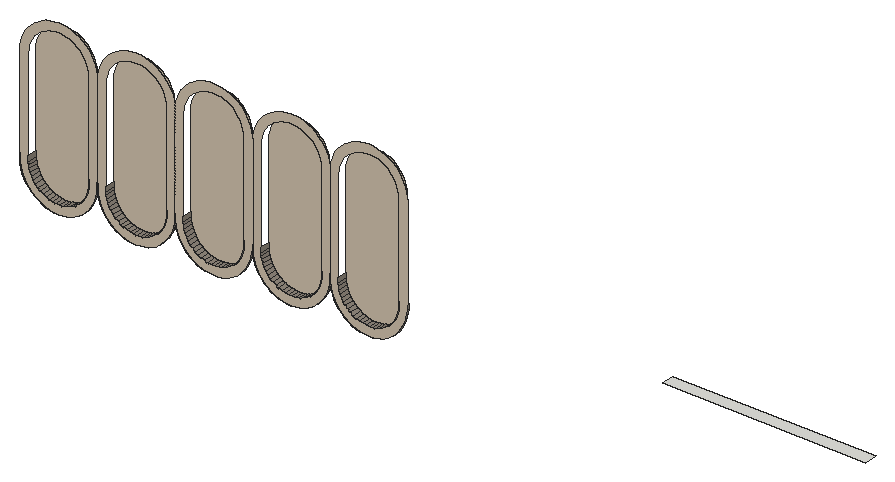
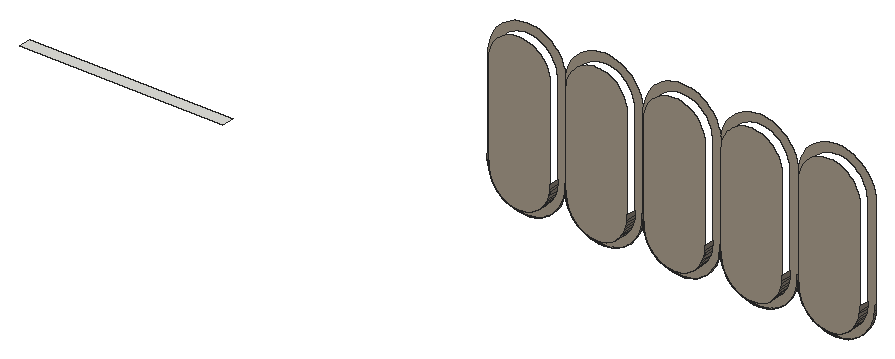
# SketchUp Ruby script. Lengths in inches.
U = 1.inch
M = Sketchup.active_model
def pt(a) = Geom::Point3d.new(a.map { |v| v * U })
def face(e, loops, mat)
  f = e.add_face(loops[0].map { |a| pt(a) })
  loops[1..].each { |l| e.add_face(l.map { |a| pt(a) }).erase! }
  f.material = f.back_material = mat if mat
  f
end
# faces: each face lists its corners as indices into pts; further lists are holes
def faces(e, pts, list, mat = nil) = list.each { |f| face(e, (f[0].is_a?(Array) ? f : [f]).map { |l| l.map { |i| pts[i] } }, mat) }
# xy, xz, yz: faces in a plane at the given z, y or x. An outline is a flat list of corners, or four numbers for a rectangle; further outlines are holes
def ring(l) = l.size == 4 ? [[l[0], l[1]], [l[2], l[1]], [l[2], l[3]], [l[0], l[3]]] : l.each_slice(2).to_a
def flat(e, list, mat, &to3) = list.each { |f| face(e, (f[0].is_a?(Array) ? f : [f]).map { |l| ring(l).map { |u, v| to3.(u, v) } }, mat) }
def xy(e, z, list, mat = nil) = flat(e, list, mat) { |x, y| [x, y, z] }
def xz(e, y, list, mat = nil) = flat(e, list, mat) { |x, z| [x, y, z] }
def yz(e, x, list, mat = nil) = flat(e, list, mat) { |y, z| [x, y, z] }
def lines(e, pts, list) = list.each { |a, b| e.add_line(pt(pts[a]), pt(pts[b])) }
# prism: a flat outline (further loops are holes) pulled along v
def prism(e, loops, v, mat = nil)
  f = face(e, loops, mat); d = Geom::Vector3d.new(v.map { |x| x * U })
  f.pushpull(f.normal.samedirection?(d) ? d.length : -d.length)
end
def box(e, o, s, mat = nil) = prism(e, [[o, [o[0] + s[0], o[1], o[2]], [o[0] + s[0], o[1] + s[1], o[2]], [o[0], o[1] + s[1], o[2]]]], [0, 0, s[2]], mat)
def at(x, y, z, deg = 0) = Geom::Transformation.translation(pt([x, y, z])) * Geom::Transformation.rotation(ORIGIN, Z_AXIS, deg.degrees)
def axes(o, x, y, z) = Geom::Transformation.new([*x, 0, *y, 0, *z, 0, *pt(o).to_a, 1])
def part(name) = M.definitions.add(name)
# library, detail: a bought-in or finely detailed component or shape, given as its bounding box
def library(name, o, s) = part(name).tap { |d| box(d.entities, o, s) }
def detail(e, o, s) = box(e.add_group.entities, o, s)
def put(e, d, t, mat = nil) = e.add_instance(d, t).tap { |i| i.material = mat if mat }
def group(e, t, mat = nil) = e.add_group.tap { |g| g.transformation = t; g.material = mat if mat }.entities
root = M.entities
M.materials.add("Heather_Band").color = [142, 133, 122]
M.materials.add("Lily_Blonde").color = [209, 194, 173]
xy(root,960.77,[[363.26,35.95,481.45,43.35]])
xz(root,3.89,[[[37.11,948.03,39.59,948.16,42.03,948.57,44.41,949.24,46.71,950.17,48.89,951.34,50.93,952.74,52.81,954.36,54.49,956.17,55.97,958.16,57.22,960.29,58.23,962.55,58.99,964.91,59.49,967.34,59.67,969.34,59.67,1026.72,59.5,1028.68,59,1031.11,58.24,1033.47,57.23,1035.73,55.98,1037.87,54.5,1039.86,52.82,1041.68,50.94,1043.3,48.9,1044.7,46.72,1045.875,44.42,1046.8,42.03,1047.47,39.59,1047.88,37.11,1048.02,34.64,1047.88,32.19,1047.47,29.81,1046.8,27.51,1045.875,25.33,1044.7,23.28,1043.3,21.41,1041.68,19.72,1039.86,18.24,1037.87,16.99,1035.73,15.98,1033.47,15.23,1031.11,14.73,1028.68,14.55,1026.72,14.55,969.34,14.74,967.34,15.23,964.91,15.99,962.55,17,960.29,18.26,958.16,19.73,956.17,21.42,954.36,23.3,952.74,25.34,951.34,27.52,950.17,29.8125,949.24,32.2,948.57,34.64,948.16],[37.11,952.88,35.17,952.99,33.25,953.3,31.38,953.83,29.58,954.56,27.86,955.48,26.26,956.58,24.79,957.85,23.46,959.28,22.3,960.84,21.32,962.51,20.52,964.29,19.93,966.14,19.54,968.05,19.4,969.5625,19.4,1026.5,19.53,1027.98,19.92,1029.88,20.51,1031.74,21.31,1033.52,22.29,1035.2,23.45,1036.76,24.78,1038.18,26.25,1039.46,27.85,1040.5625,29.57,1041.48,31.375,1042.21,33.25,1042.74,35.17,1043.06,37.11,1043.16,39.06,1043.06,40.98,1042.74,42.85,1042.21,44.66,1041.48,46.37,1040.5625,47.98,1039.46,49.45,1038.18,50.77,1036.76,51.9375,1035.2,52.92,1033.52,53.71,1031.74,54.31,1029.88,54.7,1027.98,54.83,1026.5,54.83,969.5625,54.69,968.05,54.3,966.14,53.71,964.29,52.91,962.51,51.93,960.84,50.77,959.28,49.44,957.85,47.97,956.58,46.36,955.48,44.65,954.56,42.85,953.83,40.97,953.3,39.06,952.99]]],"Lily_Blonde")
xz(root,4.02,[[[82.24,948.03,84.71,948.16,87.15,948.57,89.53,949.24,91.83,950.17,94.01,951.34,96.05,952.74,97.93,954.36,99.61,956.17,101.09,958.16,102.35,960.29,103.36,962.55,104.12,964.91,104.61,967.34,104.8,969.34,104.8,1026.72,104.62,1028.68,104.125,1031.11,103.37,1033.47,102.36,1035.73,101.1,1037.87,99.625,1039.86,97.9375,1041.68,96.0625,1043.3,94.02,1044.7,91.84,1045.875,89.54,1046.8,87.15,1047.47,84.71,1047.88,82.24,1048.02,79.76,1047.88,77.32,1047.47,74.93,1046.8,72.63,1045.875,70.45,1044.7,68.41,1043.3,66.53,1041.68,64.84,1039.86,63.37,1037.87,62.11,1035.73,61.1,1033.47,60.35,1031.11,59.85,1028.68,59.67,1026.72,59.72,1026.21,59.67,1023.73,59.67,972.28,59.72,969.8,59.67,969.34,59.86,967.34,60.36,964.91,61.11,962.55,62.125,960.29,63.38,958.16,64.86,956.17,66.54,954.36,68.42,952.74,70.46,951.34,72.64,950.17,74.9375,949.24,77.32,948.57,79.76,948.16],[82.24,952.88,80.29,952.99,78.375,953.3,76.5,953.83,74.7,954.56,72.98,955.48,71.38,956.58,69.91,957.85,68.58,959.28,67.42,960.84,66.4375,962.51,65.64,964.29,65.05,966.14,64.66,968.05,64.52,969.5625,64.52,1026.5,64.65,1027.98,65.04,1029.88,65.64,1031.74,66.43,1033.52,67.41,1035.2,68.57,1036.76,69.9,1038.18,71.37,1039.46,72.98,1040.5625,74.69,1041.48,76.5,1042.21,78.37,1042.74,80.29,1043.06,82.24,1043.16,84.18,1043.06,86.1,1042.74,87.97,1042.21,89.78,1041.48,91.49,1040.5625,93.1,1039.46,94.57,1038.18,95.9,1036.76,97.06,1035.2,98.04,1033.52,98.83,1031.74,99.43,1029.88,99.82,1027.98,99.95,1026.5,99.95,969.5625,99.8125,968.05,99.42,966.14,98.83,964.29,98.03,962.51,97.05,960.84,95.89,959.28,94.5625,957.85,93.09,956.58,91.49,955.48,89.77,954.56,87.97,953.83,86.1,953.3,84.18,952.99]],[[127.36,948.03,129.83,948.16,132.27,948.57,134.66,949.24,136.95,950.17,139.13,951.34,141.18,952.74,143.05,954.36,144.74,956.17,146.21,958.16,147.47,960.29,148.48,962.55,149.24,964.91,149.73,967.34,149.92,969.34,149.92,1026.72,149.74,1028.68,149.25,1031.11,148.49,1033.47,147.48,1035.73,146.23,1037.87,144.75,1039.86,143.0625,1041.68,141.1875,1043.3,139.14,1044.7,136.96,1045.875,134.66,1046.8,132.28,1047.47,129.83,1047.88,127.36,1048.02,124.88,1047.88,122.4375,1047.47,120.05,1046.8,117.75,1045.875,115.57,1044.7,113.53,1043.3,111.65,1041.68,109.97,1039.86,108.49,1037.87,107.24,1035.73,106.23,1033.47,105.47,1031.11,104.98,1028.68,104.8,1026.72,104.84,1026.21,104.8,1023.73,104.8,972.28,104.84,969.8,104.8,969.34,104.98,967.34,105.48,964.91,106.24,962.55,107.25,960.29,108.5,958.16,109.98,956.17,111.66,954.36,113.54,952.74,115.58,951.34,117.76,950.17,120.06,949.24,122.44,948.57,124.88,948.16],[127.36,952.88,125.41,952.99,123.5,953.3,121.625,953.83,119.82,954.56,118.11,955.48,116.5,956.58,115.03,957.85,113.7,959.28,112.54,960.84,111.56,962.51,110.77,964.29,110.17,966.14,109.78,968.05,109.64,969.5625,109.64,1026.5,109.77,1027.98,110.16,1029.88,110.76,1031.74,111.55,1033.52,112.53,1035.2,113.7,1036.76,115.02,1038.18,116.49,1039.46,118.1,1040.5625,119.8125,1041.48,121.62,1042.21,123.49,1042.74,125.41,1043.06,127.36,1043.16,129.3,1043.06,131.22,1042.74,133.1,1042.21,134.9,1041.48,136.62,1040.5625,138.22,1039.46,139.69,1038.18,141.02,1036.76,142.18,1035.2,143.16,1033.52,143.96,1031.74,144.55,1029.88,144.9375,1027.98,145.07,1026.5,145.07,969.5625,144.93,968.05,144.54,966.14,143.95,964.29,143.15,962.51,142.17,960.84,141.01,959.28,139.68,957.85,138.21,956.58,136.61,955.48,134.9,954.56,133.09,953.83,131.22,953.3,129.3,952.99]],[[172.48,948.03,174.95,948.16,177.39,948.57,179.78,949.24,182.08,950.17,184.26,951.34,186.3,952.74,188.17,954.36,189.86,956.17,191.34,958.16,192.59,960.29,193.6,962.55,194.36,964.91,194.86,967.34,195.04,969.34,195.04,1026.72,194.86,1028.68,194.37,1031.11,193.61,1033.47,192.6,1035.73,191.35,1037.87,189.87,1039.86,188.18,1041.68,186.31,1043.3,184.27,1044.7,182.08,1045.875,179.78,1046.8,177.4,1047.47,174.95,1047.88,172.48,1048.02,170,1047.88,167.56,1047.47,165.17,1046.8,162.875,1045.875,160.69,1044.7,158.65,1043.3,156.78,1041.68,155.09,1039.86,153.61,1037.87,152.36,1035.73,151.35,1033.47,150.59,1031.11,150.1,1028.68,149.92,1026.72,149.96,1026.21,149.92,1023.73,149.92,972.28,149.96,969.8,149.92,969.34,150.1,967.34,150.6,964.91,151.36,962.55,152.37,960.29,153.62,958.16,155.1,956.17,156.79,954.36,158.66,952.74,160.7,951.34,162.88,950.17,165.18,949.24,167.5625,948.57,170.01,948.16],[172.48,952.88,170.54,952.99,168.62,953.3,166.74,953.83,164.94,954.56,163.23,955.48,161.625,956.58,160.15,957.85,158.83,959.28,157.67,960.84,156.68,962.51,155.89,964.29,155.29,966.14,154.9,968.05,154.76,969.5625,154.76,1026.5,154.9,1027.98,155.28,1029.88,155.88,1031.74,156.67,1033.52,157.66,1035.2,158.82,1036.76,160.14,1038.18,161.62,1039.46,163.22,1040.5625,164.93,1041.48,166.74,1042.21,168.61,1042.74,170.53,1043.06,172.48,1043.16,174.42,1043.06,176.34,1042.74,178.22,1042.21,180.02,1041.48,181.74,1040.5625,183.34,1039.46,184.82,1038.18,186.14,1036.76,187.3,1035.2,188.29,1033.52,189.08,1031.74,189.67,1029.88,190.0625,1027.98,190.2,1026.5,190.2,969.5625,190.06,968.05,189.67,966.14,189.07,964.29,188.28,962.51,187.29,960.84,186.13,959.28,184.81,957.85,183.33,956.58,181.73,955.48,180.02,954.56,178.21,953.83,176.34,953.3,174.42,952.99]],[[217.6,948.03,220.07,948.16,222.52,948.57,224.9,949.24,227.2,950.17,229.38,951.34,231.42,952.74,233.29,954.36,234.98,956.17,236.46,958.16,237.71,960.29,238.72,962.55,239.48,964.91,239.98,967.34,240.16,969.34,240.16,1026.72,239.98,1028.68,239.49,1031.11,238.73,1033.47,237.72,1035.73,236.47,1037.87,234.99,1039.86,233.3,1041.68,231.43,1043.3,229.39,1044.7,227.2,1045.875,224.91,1046.8,222.52,1047.47,220.08,1047.88,217.6,1048.02,215.125,1047.88,212.68,1047.47,210.3,1046.8,208,1045.875,205.8125,1044.7,203.77,1043.3,201.9,1041.68,200.21,1039.86,198.73,1037.87,197.48,1035.73,196.47,1033.47,195.71,1031.11,195.22,1028.68,195.04,1026.72,195.09,1026.21,195.04,1023.73,195.04,972.28,195.08,969.8,195.04,969.34,195.22,967.34,195.72,964.91,196.48,962.55,197.49,960.29,198.74,958.16,200.22,956.17,201.91,954.36,203.78,952.74,205.82,951.34,208,950.17,210.3,949.24,212.69,948.57,215.13,948.16],[217.6,952.88,215.66,952.99,213.74,953.3,211.87,953.83,210.0625,954.56,208.35,955.48,206.75,956.58,205.27,957.85,203.95,959.28,202.79,960.84,201.8,962.51,201.01,964.29,200.41,966.14,200.02,968.05,199.88,969.5625,199.88,1026.5,200.02,1027.98,200.41,1029.88,201,1031.74,201.79,1033.52,202.78,1035.2,203.9375,1036.76,205.26,1038.18,206.74,1039.46,208.34,1040.5625,210.06,1041.48,211.86,1042.21,213.74,1042.74,215.66,1043.06,217.6,1043.16,219.54,1043.06,221.47,1042.74,223.34,1042.21,225.15,1041.48,226.86,1040.5625,228.46,1039.46,229.9375,1038.18,231.26,1036.76,232.42,1035.2,233.41,1033.52,234.2,1031.74,234.8,1029.88,235.18,1027.98,235.32,1026.5,235.32,969.5625,235.18,968.05,234.79,966.14,234.19,964.29,233.4,962.51,232.41,960.84,231.25,959.28,229.93,957.85,228.46,956.58,226.85,955.48,225.14,954.56,223.33,953.83,221.46,953.3,219.54,952.99]]],"Lily_Blonde")
xz(root,4.77,[[14.55,969.34,14.55,972.28,14.51,969.8],[59.67,969.34,59.72,969.8,59.67,972.28],[104.8,969.34,104.84,969.8,104.8,972.28],[149.92,969.34,149.96,969.8,149.92,972.28],[195.04,969.34,195.08,969.8,195.04,972.28]],"Heather_Band")
xz(root,9.67,[[37.11,952.88,39.06,952.99,40.97,953.3,42.85,953.83,44.65,954.56,46.36,955.48,47.97,956.58,49.44,957.85,50.77,959.28,51.93,960.84,52.91,962.51,53.71,964.29,54.3,966.14,54.69,968.05,54.83,969.5625,54.83,1026.5,54.7,1027.98,54.31,1029.88,53.71,1031.74,52.92,1033.52,51.9375,1035.2,50.77,1036.76,49.45,1038.18,47.98,1039.46,46.37,1040.5625,44.66,1041.48,42.85,1042.21,40.98,1042.74,39.06,1043.06,37.11,1043.16,35.17,1043.06,33.25,1042.74,31.375,1042.21,29.57,1041.48,27.85,1040.5625,26.25,1039.46,24.78,1038.18,23.45,1036.76,22.29,1035.2,21.31,1033.52,20.51,1031.74,19.92,1029.88,19.53,1027.98,19.4,1026.5,19.4,969.5625,19.54,968.05,19.93,966.14,20.52,964.29,21.32,962.51,22.3,960.84,23.46,959.28,24.79,957.85,26.26,956.58,27.86,955.48,29.58,954.56,31.38,953.83,33.25,953.3,35.17,952.99],[82.24,952.88,84.18,952.99,86.1,953.3,87.97,953.83,89.77,954.56,91.49,955.48,93.09,956.58,94.5625,957.85,95.89,959.28,97.05,960.84,98.03,962.51,98.83,964.29,99.42,966.14,99.8125,968.05,99.95,969.5625,99.95,1026.5,99.82,1027.98,99.43,1029.88,98.83,1031.74,98.04,1033.52,97.06,1035.2,95.9,1036.76,94.57,1038.18,93.1,1039.46,91.49,1040.5625,89.78,1041.48,87.97,1042.21,86.1,1042.74,84.18,1043.06,82.24,1043.16,80.29,1043.06,78.37,1042.74,76.5,1042.21,74.69,1041.48,72.98,1040.5625,71.37,1039.46,69.9,1038.18,68.57,1036.76,67.41,1035.2,66.43,1033.52,65.64,1031.74,65.04,1029.88,64.65,1027.98,64.52,1026.5,64.52,969.5625,64.66,968.05,65.05,966.14,65.64,964.29,66.4375,962.51,67.42,960.84,68.58,959.28,69.91,957.85,71.38,956.58,72.98,955.48,74.7,954.56,76.5,953.83,78.375,953.3,80.29,952.99],[127.36,952.88,129.3,952.99,131.22,953.3,133.09,953.83,134.9,954.56,136.61,955.48,138.21,956.58,139.68,957.85,141.01,959.28,142.17,960.84,143.15,962.51,143.95,964.29,144.54,966.14,144.93,968.05,145.07,969.5625,145.07,1026.5,144.9375,1027.98,144.55,1029.88,143.96,1031.74,143.16,1033.52,142.18,1035.2,141.02,1036.76,139.69,1038.18,138.22,1039.46,136.62,1040.5625,134.9,1041.48,133.1,1042.21,131.22,1042.74,129.3,1043.06,127.36,1043.16,125.41,1043.06,123.49,1042.74,121.62,1042.21,119.8125,1041.48,118.1,1040.5625,116.49,1039.46,115.02,1038.18,113.7,1036.76,112.53,1035.2,111.55,1033.52,110.76,1031.74,110.16,1029.88,109.77,1027.98,109.64,1026.5,109.64,969.5625,109.78,968.05,110.17,966.14,110.77,964.29,111.56,962.51,112.54,960.84,113.7,959.28,115.03,957.85,116.5,956.58,118.11,955.48,119.82,954.56,121.625,953.83,123.5,953.3,125.41,952.99],[172.48,952.88,174.42,952.99,176.34,953.3,178.21,953.83,180.02,954.56,181.73,955.48,183.33,956.58,184.81,957.85,186.13,959.28,187.29,960.84,188.28,962.51,189.07,964.29,189.67,966.14,190.06,968.05,190.2,969.5625,190.2,1026.5,190.0625,1027.98,189.67,1029.88,189.08,1031.74,188.29,1033.52,187.3,1035.2,186.14,1036.76,184.82,1038.18,183.34,1039.46,181.74,1040.5625,180.02,1041.48,178.22,1042.21,176.34,1042.74,174.42,1043.06,172.48,1043.16,170.53,1043.06,168.61,1042.74,166.74,1042.21,164.93,1041.48,163.22,1040.5625,161.62,1039.46,160.14,1038.18,158.82,1036.76,157.66,1035.2,156.67,1033.52,155.88,1031.74,155.28,1029.88,154.9,1027.98,154.76,1026.5,154.76,969.5625,154.9,968.05,155.29,966.14,155.89,964.29,156.68,962.51,157.67,960.84,158.83,959.28,160.15,957.85,161.625,956.58,163.23,955.48,164.94,954.56,166.74,953.83,168.62,953.3,170.54,952.99],[217.6,952.88,219.54,952.99,221.46,953.3,223.33,953.83,225.14,954.56,226.85,955.48,228.46,956.58,229.93,957.85,231.25,959.28,232.41,960.84,233.4,962.51,234.19,964.29,234.79,966.14,235.18,968.05,235.32,969.5625,235.32,1026.5,235.18,1027.98,234.8,1029.88,234.2,1031.74,233.41,1033.52,232.42,1035.2,231.26,1036.76,229.9375,1038.18,228.46,1039.46,226.86,1040.5625,225.15,1041.48,223.34,1042.21,221.47,1042.74,219.54,1043.06,217.6,1043.16,215.66,1043.06,213.74,1042.74,211.86,1042.21,210.06,1041.48,208.34,1040.5625,206.74,1039.46,205.26,1038.18,203.9375,1036.76,202.78,1035.2,201.79,1033.52,201,1031.74,200.41,1029.88,200.02,1027.98,199.88,1026.5,199.88,969.5625,200.02,968.05,200.41,966.14,201.01,964.29,201.8,962.51,202.79,960.84,203.95,959.28,205.27,957.85,206.75,956.58,208.35,955.48,210.0625,954.56,211.87,953.83,213.74,953.3,215.66,952.99]],"Lily_Blonde")
yz(root,14.55,[[3.89,969.34,4.77,972.28]],"Heather_Band")
yz(root,19.4,[[3.89,969.5625,9.67,972.28]],"Heather_Band")
yz(root,54.83,[[3.89,969.5625,9.67,972.28]],"Heather_Band")
yz(root,59.67,[[3.89,969.34,4.77,972.28]],"Heather_Band")
yz(root,64.52,[[4.02,969.5625,9.67,972.28]],"Heather_Band")
yz(root,99.95,[[4.02,969.5625,9.67,972.28]],"Heather_Band")
yz(root,104.8,[[4.02,969.34,4.77,972.28]],"Heather_Band")
yz(root,109.64,[[4.02,969.5625,9.67,972.28]],"Heather_Band")
yz(root,145.07,[[4.02,969.5625,9.67,972.28]],"Heather_Band")
yz(root,149.92,[[4.02,969.34,4.77,972.28]],"Heather_Band")
yz(root,154.76,[[4.02,969.5625,9.67,972.28]],"Heather_Band")
yz(root,190.2,[[4.02,969.5625,9.67,972.28]],"Heather_Band")
yz(root,195.04,[[4.02,969.34,4.77,972.28]],"Heather_Band")
yz(root,199.88,[[4.02,969.5625,9.67,972.28]],"Heather_Band")
yz(root,235.32,[[4.02,969.5625,9.67,972.28]],"Heather_Band")
yz(root,240.16,[[4.02,969.34,4.77,972.28]],"Heather_Band")
p = [[34.64,4.77,948.16],[37.11,4.77,948.03],[37.11,3.89,948.03],[34.64,3.89,948.16],[39.59,4.77,948.16],[39.59,3.89,948.16],
  [79.76,4.77,948.16],[82.24,4.77,948.03],[82.24,4.02,948.03],[79.76,4.02,948.16],[84.71,4.77,948.16],[84.71,4.02,948.16],
  [124.88,4.77,948.16],[127.36,4.77,948.03],[127.36,4.02,948.03],[124.88,4.02,948.16],[129.83,4.77,948.16],[129.83,4.02,948.16],
  [170.01,4.77,948.16],[172.48,4.77,948.03],[172.48,4.02,948.03],[170.01,4.02,948.16],[174.95,4.77,948.16],[174.95,4.02,948.16],
  [215.13,4.77,948.16],[217.6,4.77,948.03],[217.6,4.02,948.03],[215.13,4.02,948.16],[220.07,4.77,948.16],[220.07,4.02,948.16],
  [32.2,4.77,948.57],[32.2,3.89,948.57],[42.03,4.77,948.57],[42.03,3.89,948.57],[77.32,4.77,948.57],[77.32,4.02,948.57],
  [87.15,4.77,948.57],[87.15,4.02,948.57],[122.44,4.77,948.57],[122.44,4.02,948.57],[132.27,4.77,948.57],[132.27,4.02,948.57],
  [167.5625,4.77,948.57],[167.5625,4.02,948.57],[177.39,4.77,948.57],[177.39,4.02,948.57],[212.69,4.77,948.57],[212.69,4.02,948.57],
  [222.52,4.77,948.57],[222.52,4.02,948.57],[29.8125,4.77,949.24],[29.8125,3.89,949.24],[44.41,4.77,949.24],[44.41,3.89,949.24],
  [74.9375,4.77,949.24],[74.9375,4.02,949.24],[89.53,4.77,949.24],[89.53,4.02,949.24],[120.06,4.77,949.24],[120.06,4.02,949.24],
  [134.66,4.77,949.24],[134.66,4.02,949.24],[165.18,4.77,949.24],[165.18,4.02,949.24],[179.78,4.77,949.24],[179.78,4.02,949.24],
  [210.3,4.77,949.24],[210.3,4.02,949.24],[224.9,4.77,949.24],[224.9,4.02,949.24],[27.52,4.77,950.17],[27.52,3.89,950.17],
  [46.71,4.77,950.17],[46.71,3.89,950.17],[72.64,4.77,950.17],[72.64,4.02,950.17],[91.83,4.77,950.17],[91.83,4.02,950.17],
  [117.76,4.77,950.17],[117.76,4.02,950.17],[136.95,4.77,950.17],[136.95,4.02,950.17],[162.88,4.77,950.17],[162.88,4.02,950.17],
  [182.08,4.77,950.17],[182.08,4.02,950.17],[208,4.77,950.17],[208,4.02,950.17],[227.2,4.77,950.17],[227.2,4.02,950.17],
  [25.34,4.77,951.34],[25.34,3.89,951.34],[48.89,4.77,951.34],[48.89,3.89,951.34],[70.46,4.77,951.34],[70.46,4.02,951.34],
  [94.01,4.77,951.34],[94.01,4.02,951.34],[115.58,4.77,951.34],[115.58,4.02,951.34],[139.13,4.77,951.34],[139.13,4.02,951.34],
  [160.7,4.77,951.34],[160.7,4.02,951.34],[184.26,4.77,951.34],[184.26,4.02,951.34],[205.82,4.77,951.34],[205.82,4.02,951.34],
  [229.38,4.77,951.34],[229.38,4.02,951.34],[23.3,4.77,952.74],[23.3,3.89,952.74],[50.93,4.77,952.74],[50.93,3.89,952.74],
  [68.42,4.77,952.74],[68.42,4.02,952.74],[96.05,4.77,952.74],[96.05,4.02,952.74],[113.54,4.77,952.74],[113.54,4.02,952.74],
  [141.18,4.77,952.74],[141.18,4.02,952.74],[158.66,4.77,952.74],[158.66,4.02,952.74],[186.3,4.77,952.74],[186.3,4.02,952.74],
  [203.78,4.77,952.74],[203.78,4.02,952.74],[231.42,4.77,952.74],[231.42,4.02,952.74],[21.42,4.77,954.36],[21.42,3.89,954.36],
  [52.81,4.77,954.36],[52.81,3.89,954.36],[66.54,4.77,954.36],[66.54,4.02,954.36],[97.93,4.77,954.36],[97.93,4.02,954.36],
  [111.66,4.77,954.36],[111.66,4.02,954.36],[143.05,4.77,954.36],[143.05,4.02,954.36],[156.79,4.77,954.36],[156.79,4.02,954.36],
  [188.17,4.77,954.36],[188.17,4.02,954.36],[201.91,4.77,954.36],[201.91,4.02,954.36],[233.29,4.77,954.36],[233.29,4.02,954.36],
  [35.17,9.67,952.99],[35.17,3.89,952.99],[37.11,3.89,952.88],[37.11,9.67,952.88],[39.06,3.89,952.99],[39.06,9.67,952.99],
  [80.29,9.67,952.99],[80.29,4.02,952.99],[82.24,4.02,952.88],[82.24,9.67,952.88],[84.18,4.02,952.99],[84.18,9.67,952.99],
  [125.41,9.67,952.99],[125.41,4.02,952.99],[127.36,4.02,952.88],[127.36,9.67,952.88],[129.3,4.02,952.99],[129.3,9.67,952.99],
  [170.54,9.67,952.99],[170.54,4.02,952.99],[172.48,4.02,952.88],[172.48,9.67,952.88],[174.42,4.02,952.99],[174.42,9.67,952.99],
  [215.66,9.67,952.99],[215.66,4.02,952.99],[217.6,4.02,952.88],[217.6,9.67,952.88],[219.54,4.02,952.99],[219.54,9.67,952.99],
  [33.25,9.67,953.3],[33.25,3.89,953.3],[40.97,3.89,953.3],[40.97,9.67,953.3],[78.375,9.67,953.3],[78.375,4.02,953.3],
  [86.1,4.02,953.3],[86.1,9.67,953.3],[123.5,9.67,953.3],[123.5,4.02,953.3],[131.22,4.02,953.3],[131.22,9.67,953.3],
  [168.62,9.67,953.3],[168.62,4.02,953.3],[176.34,4.02,953.3],[176.34,9.67,953.3],[213.74,9.67,953.3],[213.74,4.02,953.3],
  [221.46,4.02,953.3],[221.46,9.67,953.3],[31.38,9.67,953.83],[31.38,3.89,953.83],[42.85,3.89,953.83],[42.85,9.67,953.83],
  [76.5,9.67,953.83],[76.5,4.02,953.83],[87.97,4.02,953.83],[87.97,9.67,953.83],[121.625,9.67,953.83],[121.625,4.02,953.83],
  [133.09,4.02,953.83],[133.09,9.67,953.83],[166.74,9.67,953.83],[166.74,4.02,953.83],[178.21,4.02,953.83],[178.21,9.67,953.83],
  [211.87,9.67,953.83],[211.87,4.02,953.83],[223.33,4.02,953.83],[223.33,9.67,953.83],[29.58,9.67,954.56],[29.58,3.89,954.56],
  [44.65,3.89,954.56],[44.65,9.67,954.56],[74.7,9.67,954.56],[74.7,4.02,954.56],[89.77,4.02,954.56],[89.77,9.67,954.56],
  [119.82,9.67,954.56],[119.82,4.02,954.56],[134.9,4.02,954.56],[134.9,9.67,954.56],[164.94,9.67,954.56],[164.94,4.02,954.56],
  [180.02,4.02,954.56],[180.02,9.67,954.56],[210.0625,9.67,954.56],[210.0625,4.02,954.56],[225.14,4.02,954.56],[225.14,9.67,954.56],
  [19.73,4.77,956.17],[19.73,3.89,956.17],[54.49,4.77,956.17],[54.49,3.89,956.17],[64.86,4.77,956.17],[64.86,4.02,956.17],
  [99.61,4.77,956.17],[99.61,4.02,956.17],[109.98,4.77,956.17],[109.98,4.02,956.17],[144.74,4.77,956.17],[144.74,4.02,956.17],
  [155.1,4.77,956.17],[155.1,4.02,956.17],[189.86,4.77,956.17],[189.86,4.02,956.17],[200.22,4.77,956.17],[200.22,4.02,956.17],
  [234.98,4.77,956.17],[234.98,4.02,956.17],[27.86,9.67,955.48],[27.86,3.89,955.48],[46.36,3.89,955.48],[46.36,9.67,955.48],
  [72.98,9.67,955.48],[72.98,4.02,955.48],[91.49,4.02,955.48],[91.49,9.67,955.48],[118.11,9.67,955.48],[118.11,4.02,955.48],
  [136.61,4.02,955.48],[136.61,9.67,955.48],[163.23,9.67,955.48],[163.23,4.02,955.48],[181.73,4.02,955.48],[181.73,9.67,955.48],
  [208.35,9.67,955.48],[208.35,4.02,955.48],[226.85,4.02,955.48],[226.85,9.67,955.48],[26.26,9.67,956.58],[26.26,3.89,956.58],
  [47.97,3.89,956.58],[47.97,9.67,956.58],[71.38,9.67,956.58],[71.38,4.02,956.58],[93.09,4.02,956.58],[93.09,9.67,956.58],
  [116.5,9.67,956.58],[116.5,4.02,956.58],[138.21,4.02,956.58],[138.21,9.67,956.58],[161.625,9.67,956.58],[161.625,4.02,956.58],
  [183.33,4.02,956.58],[183.33,9.67,956.58],[206.75,9.67,956.58],[206.75,4.02,956.58],[228.46,4.02,956.58],[228.46,9.67,956.58],
  [18.26,4.77,958.16],[18.26,3.89,958.16],[55.97,4.77,958.16],[55.97,3.89,958.16],[63.38,4.77,958.16],[63.38,4.02,958.16],
  [101.09,4.77,958.16],[101.09,4.02,958.16],[108.5,4.77,958.16],[108.5,4.02,958.16],[146.21,4.77,958.16],[146.21,4.02,958.16],
  [153.62,4.77,958.16],[153.62,4.02,958.16],[191.34,4.77,958.16],[191.34,4.02,958.16],[198.74,4.77,958.16],[198.74,4.02,958.16],
  [236.46,4.77,958.16],[236.46,4.02,958.16],[24.79,9.67,957.85],[24.79,3.89,957.85],[49.44,3.89,957.85],[49.44,9.67,957.85],
  [69.91,9.67,957.85],[69.91,4.02,957.85],[94.5625,4.02,957.85],[94.5625,9.67,957.85],[115.03,9.67,957.85],[115.03,4.02,957.85],
  [139.68,4.02,957.85],[139.68,9.67,957.85],[160.15,9.67,957.85],[160.15,4.02,957.85],[184.81,4.02,957.85],[184.81,9.67,957.85],
  [205.27,9.67,957.85],[205.27,4.02,957.85],[229.93,4.02,957.85],[229.93,9.67,957.85],[23.46,9.67,959.28],[23.46,3.89,959.28],
  [50.77,3.89,959.28],[50.77,9.67,959.28],[68.58,9.67,959.28],[68.58,4.02,959.28],[95.89,4.02,959.28],[95.89,9.67,959.28],
  [113.7,9.67,959.28],[113.7,4.02,959.28],[141.01,4.02,959.28],[141.01,9.67,959.28],[158.83,9.67,959.28],[158.83,4.02,959.28],
  [186.13,4.02,959.28],[186.13,9.67,959.28],[203.95,9.67,959.28],[203.95,4.02,959.28],[231.25,4.02,959.28],[231.25,9.67,959.28],
  [17,4.77,960.29],[17,3.89,960.29],[57.22,4.77,960.29],[57.22,3.89,960.29],[62.125,4.77,960.29],[62.125,4.02,960.29],
  [102.35,4.77,960.29],[102.35,4.02,960.29],[107.25,4.77,960.29],[107.25,4.02,960.29],[147.47,4.77,960.29],[147.47,4.02,960.29],
  [152.37,4.77,960.29],[152.37,4.02,960.29],[192.59,4.77,960.29],[192.59,4.02,960.29],[197.49,4.77,960.29],[197.49,4.02,960.29],
  [237.71,4.77,960.29],[237.71,4.02,960.29],[22.3,9.67,960.84],[22.3,3.89,960.84],[51.93,3.89,960.84],[51.93,9.67,960.84],
  [67.42,9.67,960.84],[67.42,4.02,960.84],[97.05,4.02,960.84],[97.05,9.67,960.84],[112.54,9.67,960.84],[112.54,4.02,960.84],
  [142.17,4.02,960.84],[142.17,9.67,960.84],[157.67,9.67,960.84],[157.67,4.02,960.84],[187.29,4.02,960.84],[187.29,9.67,960.84],
  [202.79,9.67,960.84],[202.79,4.02,960.84],[232.41,4.02,960.84],[232.41,9.67,960.84],[15.99,4.77,962.55],[15.99,3.89,962.55],
  [58.23,4.77,962.55],[58.23,3.89,962.55],[61.11,4.77,962.55],[61.11,4.02,962.55],[103.36,4.77,962.55],[103.36,4.02,962.55],
  [106.24,4.77,962.55],[106.24,4.02,962.55],[148.48,4.77,962.55],[148.48,4.02,962.55],[151.36,4.77,962.55],[151.36,4.02,962.55],
  [193.6,4.77,962.55],[193.6,4.02,962.55],[196.48,4.77,962.55],[196.48,4.02,962.55],[238.72,4.77,962.55],[238.72,4.02,962.55],
  [21.32,9.67,962.51],[21.32,3.89,962.51],[52.91,3.89,962.51],[52.91,9.67,962.51],[66.4375,9.67,962.51],[66.4375,4.02,962.51],
  [98.03,4.02,962.51],[98.03,9.67,962.51],[111.56,9.67,962.51],[111.56,4.02,962.51],[143.15,4.02,962.51],[143.15,9.67,962.51],
  [156.68,9.67,962.51],[156.68,4.02,962.51],[188.28,4.02,962.51],[188.28,9.67,962.51],[201.8,9.67,962.51],[201.8,4.02,962.51],
  [233.4,4.02,962.51],[233.4,9.67,962.51],[20.52,9.67,964.29],[20.52,3.89,964.29],[53.71,3.89,964.29],[53.71,9.67,964.29],
  [65.64,9.67,964.29],[65.64,4.02,964.29],[98.83,4.02,964.29],[98.83,9.67,964.29],[110.77,9.67,964.29],[110.77,4.02,964.29],
  [143.95,4.02,964.29],[143.95,9.67,964.29],[155.89,9.67,964.29],[155.89,4.02,964.29],[189.07,4.02,964.29],[189.07,9.67,964.29],
  [201.01,9.67,964.29],[201.01,4.02,964.29],[234.19,4.02,964.29],[234.19,9.67,964.29],[15.23,4.77,964.91],[15.23,3.89,964.91],
  [58.99,4.77,964.91],[58.99,3.89,964.91],[60.36,4.77,964.91],[60.36,4.02,964.91],[104.12,4.77,964.91],[104.12,4.02,964.91],
  [105.48,4.77,964.91],[105.48,4.02,964.91],[149.24,4.77,964.91],[149.24,4.02,964.91],[150.6,4.77,964.91],[150.6,4.02,964.91],
  [194.36,4.77,964.91],[194.36,4.02,964.91],[195.72,4.77,964.91],[195.72,4.02,964.91],[239.48,4.77,964.91],[239.48,4.02,964.91],
  [19.93,9.67,966.14],[19.93,3.89,966.14],[54.3,3.89,966.14],[54.3,9.67,966.14],[65.05,9.67,966.14],[65.05,4.02,966.14],
  [99.42,4.02,966.14],[99.42,9.67,966.14],[110.17,9.67,966.14],[110.17,4.02,966.14],[144.54,4.02,966.14],[144.54,9.67,966.14],
  [155.29,9.67,966.14],[155.29,4.02,966.14],[189.67,4.02,966.14],[189.67,9.67,966.14],[200.41,9.67,966.14],[200.41,4.02,966.14],
  [234.79,4.02,966.14],[234.79,9.67,966.14],[14.74,4.77,967.34],[14.74,3.89,967.34],[59.49,4.77,967.34],[59.49,3.89,967.34],
  [59.86,4.77,967.34],[59.86,4.02,967.34],[104.61,4.77,967.34],[104.61,4.02,967.34],[104.98,4.77,967.34],[104.98,4.02,967.34],
  [149.73,4.77,967.34],[149.73,4.02,967.34],[150.1,4.77,967.34],[150.1,4.02,967.34],[194.86,4.77,967.34],[194.86,4.02,967.34],
  [195.22,4.77,967.34],[195.22,4.02,967.34],[239.98,4.77,967.34],[239.98,4.02,967.34],[19.54,9.67,968.05],[19.54,3.89,968.05],
  [54.69,3.89,968.05],[54.69,9.67,968.05],[64.66,9.67,968.05],[64.66,4.02,968.05],[99.8125,4.02,968.05],[99.8125,9.67,968.05],
  [109.78,9.67,968.05],[109.78,4.02,968.05],[144.93,4.02,968.05],[144.93,9.67,968.05],[154.9,9.67,968.05],[154.9,4.02,968.05],
  [190.06,4.02,968.05],[190.06,9.67,968.05],[200.02,9.67,968.05],[200.02,4.02,968.05],[235.18,4.02,968.05],[235.18,9.67,968.05],
  [14.55,4.77,969.34],[14.55,3.89,969.34],[59.67,4.77,969.34],[59.67,4.02,969.34],[59.67,3.89,969.34],[104.8,4.77,969.34],
  [104.8,4.02,969.34],[149.92,4.77,969.34],[149.92,4.02,969.34],[195.04,4.77,969.34],[195.04,4.02,969.34],[240.16,4.77,969.34],
  [240.16,4.02,969.34],[19.4,9.67,969.5625],[19.4,3.89,969.5625],[54.83,3.89,969.5625],[54.83,9.67,969.5625],[64.52,9.67,969.5625],
  [64.52,4.02,969.5625],[99.95,4.02,969.5625],[99.95,9.67,969.5625],[109.64,9.67,969.5625],[109.64,4.02,969.5625],[145.07,4.02,969.5625],
  [145.07,9.67,969.5625],[154.76,9.67,969.5625],[154.76,4.02,969.5625],[190.2,4.02,969.5625],[190.2,9.67,969.5625],[199.88,9.67,969.5625],
  [199.88,4.02,969.5625],[235.32,4.02,969.5625],[235.32,9.67,969.5625],[59.72,4.77,969.8],[59.72,4.02,969.8],[104.84,4.77,969.8],
  [104.84,4.02,969.8],[149.96,4.77,969.8],[149.96,4.02,969.8],[195.08,4.77,969.8],[195.08,4.02,969.8],[59.67,4.77,972.28],
  [59.67,4.02,972.28],[104.8,4.77,972.28],[104.8,4.02,972.28],[149.92,4.77,972.28],[149.92,4.02,972.28],[195.04,4.77,972.28],
  [195.04,4.02,972.28]]
faces(root,p,[[0,1,2,3],[1,4,5,2],[6,7,8,9],[7,10,11,8],[12,13,14,15],[13,16,17,14],[18,19,20,21],[19,22,23,20],
  [24,25,26,27],[25,28,29,26],[30,0,3,31],[4,32,33,5],[34,6,9,35],[10,36,37,11],[38,12,15,39],[16,40,41,17],
  [42,18,21,43],[22,44,45,23],[46,24,27,47],[28,48,49,29],[50,30,31,51],[32,52,53,33],[54,34,35,55],[36,56,57,37],
  [58,38,39,59],[40,60,61,41],[62,42,43,63],[44,64,65,45],[66,46,47,67],[48,68,69,49],[70,50,51,71],[52,72,73,53],
  [74,54,55,75],[56,76,77,57],[78,58,59,79],[60,80,81,61],[82,62,63,83],[64,84,85,65],[86,66,67,87],[68,88,89,69],
  [90,70,71,91],[72,92,93,73],[94,74,75,95],[76,96,97,77],[98,78,79,99],[80,100,101,81],[102,82,83,103],[84,104,105,85],
  [106,86,87,107],[88,108,109,89],[110,90,91,111],[92,112,113,93],[114,94,95,115],[96,116,117,97],[118,98,99,119],[100,120,121,101],
  [122,102,103,123],[104,124,125,105],[126,106,107,127],[108,128,129,109],[130,110,111,131],[112,132,133,113],[134,114,115,135],[116,136,137,117],
  [138,118,119,139],[120,140,141,121],[142,122,123,143],[124,144,145,125],[146,126,127,147],[128,148,149,129],[150,151,152,153],[153,152,154,155],
  [156,157,158,159],[159,158,160,161],[162,163,164,165],[165,164,166,167],[168,169,170,171],[171,170,172,173],[174,175,176,177],[177,176,178,179],
  [180,181,151,150],[155,154,182,183],[184,185,157,156],[161,160,186,187],[188,189,163,162],[167,166,190,191],[192,193,169,168],[173,172,194,195],
  [196,197,175,174],[179,178,198,199],[200,201,181,180],[183,182,202,203],[204,205,185,184],[187,186,206,207],[208,209,189,188],[191,190,210,211],
  [212,213,193,192],[195,194,214,215],[216,217,197,196],[199,198,218,219],[220,221,201,200],[203,202,222,223],[224,225,205,204],[207,206,226,227],
  [228,229,209,208],[211,210,230,231],[232,233,213,212],[215,214,234,235],[236,237,217,216],[219,218,238,239],[240,130,131,241],[132,242,243,133],
  [244,134,135,245],[136,246,247,137],[248,138,139,249],[140,250,251,141],[252,142,143,253],[144,254,255,145],[256,146,147,257],[148,258,259,149],
  [260,261,221,220],[223,222,262,263],[264,265,225,224],[227,226,266,267],[268,269,229,228],[231,230,270,271],[272,273,233,232],[235,234,274,275],
  [276,277,237,236],[239,238,278,279],[280,281,261,260],[263,262,282,283],[284,285,265,264],[267,266,286,287],[288,289,269,268],[271,270,290,291],
  [292,293,273,272],[275,274,294,295],[296,297,277,276],[279,278,298,299],[300,240,241,301],[242,302,303,243],[304,244,245,305],[246,306,307,247],
  [308,248,249,309],[250,310,311,251],[312,252,253,313],[254,314,315,255],[316,256,257,317],[258,318,319,259],[320,321,281,280],[283,282,322,323],
  [324,325,285,284],[287,286,326,327],[328,329,289,288],[291,290,330,331],[332,333,293,292],[295,294,334,335],[336,337,297,296],[299,298,338,339],
  [340,341,321,320],[323,322,342,343],[344,345,325,324],[327,326,346,347],[348,349,329,328],[331,330,350,351],[352,353,333,332],[335,334,354,355],
  [356,357,337,336],[339,338,358,359],[360,300,301,361],[302,362,363,303],[364,304,305,365],[306,366,367,307],[368,308,309,369],[310,370,371,311],
  [372,312,313,373],[314,374,375,315],[376,316,317,377],[318,378,379,319],[380,381,341,340],[343,342,382,383],[384,385,345,344],[347,346,386,387],
  [388,389,349,348],[351,350,390,391],[392,393,353,352],[355,354,394,395],[396,397,357,356],[359,358,398,399],[400,360,361,401],[362,402,403,363],
  [404,364,365,405],[366,406,407,367],[408,368,369,409],[370,410,411,371],[412,372,373,413],[374,414,415,375],[416,376,377,417],[378,418,419,379],
  [420,421,381,380],[383,382,422,423],[424,425,385,384],[387,386,426,427],[428,429,389,388],[391,390,430,431],[432,433,393,392],[395,394,434,435],
  [436,437,397,396],[399,398,438,439],[440,441,421,420],[423,422,442,443],[444,445,425,424],[427,426,446,447],[448,449,429,428],[431,430,450,451],
  [452,453,433,432],[435,434,454,455],[456,457,437,436],[439,438,458,459],[460,400,401,461],[402,462,463,403],[464,404,405,465],[406,466,467,407],
  [468,408,409,469],[410,470,471,411],[472,412,413,473],[414,474,475,415],[476,416,417,477],[418,478,479,419],[480,481,441,440],[443,442,482,483],
  [484,485,445,444],[447,446,486,487],[488,489,449,448],[451,450,490,491],[492,493,453,452],[455,454,494,495],[496,497,457,456],[459,458,498,499],
  [500,460,461,501],[462,502,503,463],[504,464,465,505],[466,506,507,467],[508,468,469,509],[470,510,511,471],[512,472,473,513],[474,514,515,475],
  [516,476,477,517],[478,518,519,479],[520,521,481,480],[483,482,522,523],[524,525,485,484],[487,486,526,527],[528,529,489,488],[491,490,530,531],
  [532,533,493,492],[495,494,534,535],[536,537,497,496],[499,498,538,539],[540,500,501,541],[502,542,543,544,503],[542,504,505,543],[506,545,546,507],
  [545,508,509,546],[510,547,548,511],[547,512,513,548],[514,549,550,515],[549,516,517,550],[518,551,552,519],[553,554,521,520],[523,522,555,556],
  [557,558,525,524],[527,526,559,560],[561,562,529,528],[531,530,563,564],[565,566,533,532],[535,534,567,568],[569,570,537,536],[539,538,571,572],
  [573,542,543,574],[575,545,546,576],[577,547,548,578],[579,549,550,580],[581,573,574,582],[583,575,576,584],[585,577,578,586],[587,579,580,588]],"Heather_Band")
